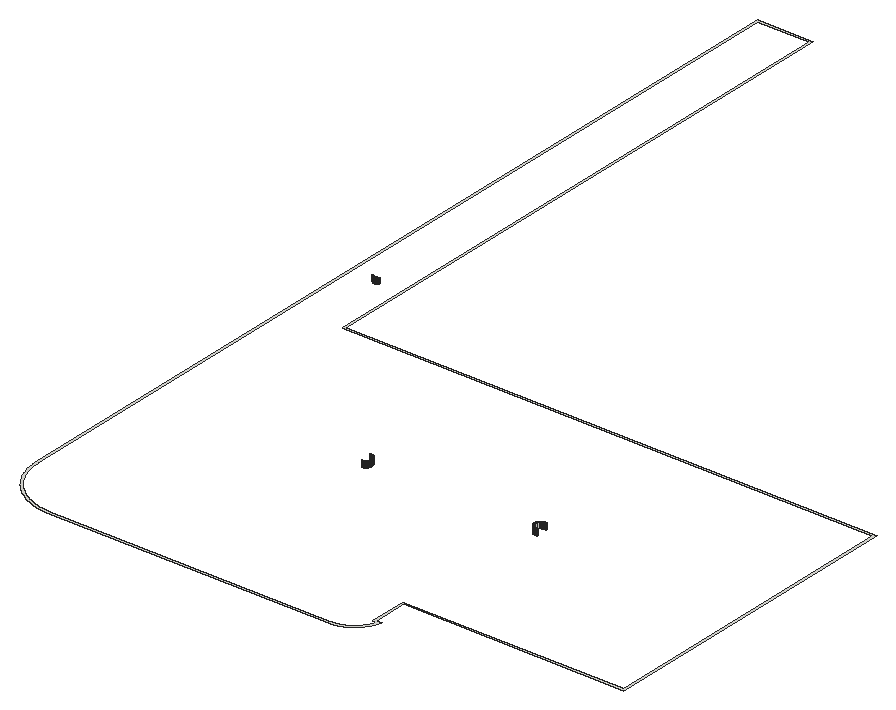
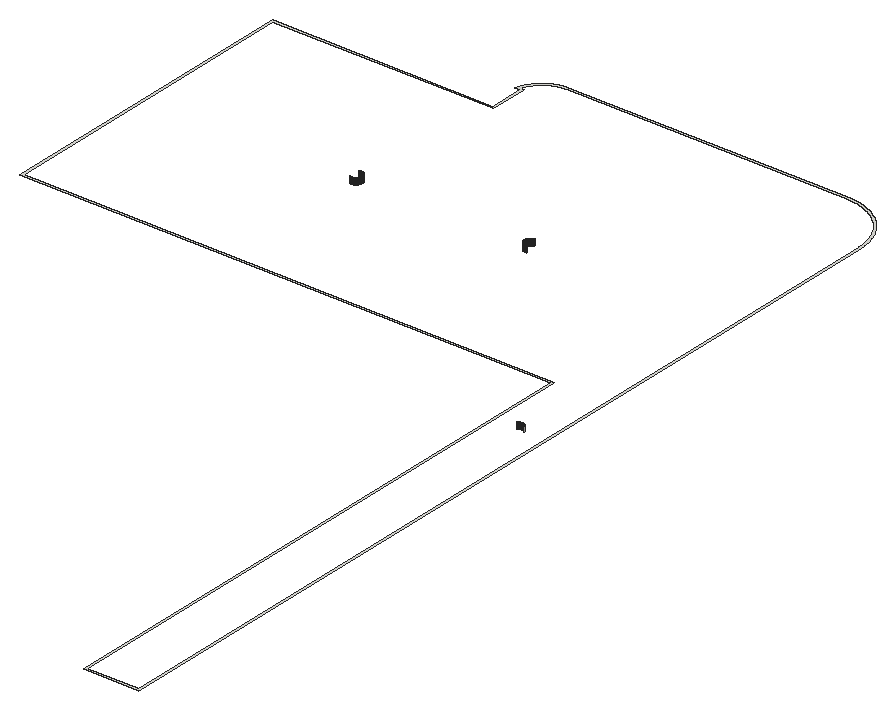
# SketchUp Ruby script. Lengths in inches.
U = 1.inch
M = Sketchup.active_model
def pt(a) = Geom::Point3d.new(a.map { |v| v * U })
def face(e, loops, mat)
  f = e.add_face(loops[0].map { |a| pt(a) })
  loops[1..].each { |l| e.add_face(l.map { |a| pt(a) }).erase! }
  f.material = f.back_material = mat if mat
  f
end
# faces: each face lists its corners as indices into pts; further lists are holes
def faces(e, pts, list, mat = nil) = list.each { |f| face(e, (f[0].is_a?(Array) ? f : [f]).map { |l| l.map { |i| pts[i] } }, mat) }
# xy, xz, yz: faces in a plane at the given z, y or x. An outline is a flat list of corners, or four numbers for a rectangle; further outlines are holes
def ring(l) = l.size == 4 ? [[l[0], l[1]], [l[2], l[1]], [l[2], l[3]], [l[0], l[3]]] : l.each_slice(2).to_a
def flat(e, list, mat, &to3) = list.each { |f| face(e, (f[0].is_a?(Array) ? f : [f]).map { |l| ring(l).map { |u, v| to3.(u, v) } }, mat) }
def xy(e, z, list, mat = nil) = flat(e, list, mat) { |x, y| [x, y, z] }
def xz(e, y, list, mat = nil) = flat(e, list, mat) { |x, z| [x, y, z] }
def yz(e, x, list, mat = nil) = flat(e, list, mat) { |y, z| [x, y, z] }
def lines(e, pts, list) = list.each { |a, b| e.add_line(pt(pts[a]), pt(pts[b])) }
# prism: a flat outline (further loops are holes) pulled along v
def prism(e, loops, v, mat = nil)
  f = face(e, loops, mat); d = Geom::Vector3d.new(v.map { |x| x * U })
  f.pushpull(f.normal.samedirection?(d) ? d.length : -d.length)
end
def box(e, o, s, mat = nil) = prism(e, [[o, [o[0] + s[0], o[1], o[2]], [o[0] + s[0], o[1] + s[1], o[2]], [o[0], o[1] + s[1], o[2]]]], [0, 0, s[2]], mat)
def at(x, y, z, deg = 0) = Geom::Transformation.translation(pt([x, y, z])) * Geom::Transformation.rotation(ORIGIN, Z_AXIS, deg.degrees)
def axes(o, x, y, z) = Geom::Transformation.new([*x, 0, *y, 0, *z, 0, *pt(o).to_a, 1])
def part(name) = M.definitions.add(name)
# library, detail: a bought-in or finely detailed component or shape, given as its bounding box
def library(name, o, s) = part(name).tap { |d| box(d.entities, o, s) }
def detail(e, o, s) = box(e.add_group.entities, o, s)
def put(e, d, t, mat = nil) = e.add_instance(d, t).tap { |i| i.material = mat if mat }
def group(e, t, mat = nil) = e.add_group.tap { |g| g.transformation = t; g.material = mat if mat }.entities
root = M.entities
xy(root,258.5,[[[43.62,68,42.86,68.02,42.48,68.04,42.1,68.0625,41.72,68.09,41.35,68.12,40.59,68.2,40.21,68.25,39.84,68.3,39.46,68.36,39.09,68.42,38.72,68.49,38.34,68.56,37.97,68.63,37.6,68.72,37.23,68.8,36.86,68.89,36.49,68.99,36.13,69.09,35.76,69.19,35.4,69.3,34.32,69.66,33.96,69.79,33.61,69.93,33.25,70.06,32.2,70.51,31.86,70.66,31.52,70.83,31.17,70.99,30.83,71.16,30.5,71.34,30.16,71.51,29.17,72.08,28.85,72.27,28.53,72.47,27.57,73.1,26.95,73.54,26.65,73.76,26.35,73.99,26.05,74.23,25.75,74.46,25.46,74.7,24.88,75.2,24.6,75.45,24.31,75.7,24.04,75.96,23.76,76.23,23.49,76.49,23.23,76.76,22.96,77.04,22.7,77.31,22.45,77.6,22.2,77.88,21.7,78.46,21.46,78.75,21.23,79.05,20.99,79.35,20.76,79.65,20.54,79.95,20.1,80.57,19.47,81.53,19.27,81.85,19.08,82.17,18.51,83.16,18.34,83.5,18.16,83.83,17.99,84.17,17.83,84.52,17.66,84.86,17.51,85.2,17.06,86.25,16.93,86.61,16.79,86.96,16.66,87.32,16.3,88.4,16.19,88.76,16.09,89.13,15.99,89.49,15.89,89.86,15.8,90.23,15.72,90.6,15.63,90.97,15.56,91.34,15.49,91.72,15.42,92.09,15.36,92.46,15.3,92.84,15.25,93.21,15.2,93.59,15.12,94.35,15.09,94.72,15.0625,95.1,15.04,95.48,15.02,95.86,15,96.62,15,551,43,551,43,257,310,257,310,98,199,98,199,81,201.52,81,201.48,80.82,201.42,80.6,201.36,80.39,201.3,80.17,201.24,79.96,201.1,79.54,201.02,79.33,200.95,79.12,200.71,78.49,200.53,78.09,200.4375,77.88,200.34,77.68,200.25,77.48,200.15,77.28,200.04,77.08,199.94,76.89,199.83,76.69,199.61,76.31,199.49,76.12,199.38,75.93,199.26,75.74,199.13,75.56,199.01,75.37,198.88,75.1875,198.75,75.01,198.49,74.65,198.35,74.48,198.21,74.3,197.93,73.96,197.78,73.79,197.48,73.46,197.18,73.14,196.86,72.82,196.54,72.52,196.21,72.22,196.04,72.07,195.7,71.79,195.52,71.65,195.35,71.51,194.99,71.25,194.8125,71.12,194.63,70.99,194.44,70.87,194.26,70.74,194.07,70.62,193.88,70.51,193.69,70.39,193.31,70.17,193.11,70.06,192.92,69.96,192.72,69.85,192.52,69.75,192.32,69.66,192.12,69.5625,191.91,69.47,191.51,69.29,190.88,69.05,190.67,68.98,190.46,68.9,190.04,68.76,189.83,68.7,189.61,68.64,189.4,68.58,189.18,68.52,188.97,68.47,188.53,68.37,188.32,68.33,188.1,68.28,187.88,68.25,187.66,68.21,187.4375,68.18,187.22,68.15,186.78,68.09,186.56,68.07,186.33,68.05,186.11,68.04,185.89,68.02,185.67,68.01,185.45,68.01,185.22,68],[43.63,69,185.21,69,185.42,69.01,185.63,69.01,186.05,69.03,186.26,69.05,186.46,69.07,186.88,69.11,187.3,69.17,187.5,69.2,187.71,69.23,187.92,69.27,188.12,69.31,188.33,69.35,188.53,69.39,188.74,69.44,188.9375,69.49,189.14,69.55,189.34,69.6,189.94,69.78,190.54,69.99,190.73,70.0625,190.93,70.14,191.12,70.22,191.32,70.3,191.51,70.38,192.08,70.65,192.26,70.74,192.45,70.84,192.63,70.9375,192.82,71.04,193,71.14,193.54,71.47,193.71,71.58,193.89,71.7,194.0625,71.8125,194.23,71.93,194.4,72.06,194.57,72.18,194.91,72.44,195.39,72.83,195.71,73.11,196.01,73.39,196.16,73.54,196.3125,73.6875,196.46,73.84,196.61,73.99,196.89,74.29,197.17,74.61,197.56,75.09,197.82,75.43,197.94,75.6,198.07,75.77,198.1875,75.9375,198.3,76.11,198.42,76.29,198.53,76.46,198.86,77,198.96,77.18,199.0625,77.37,199.16,77.55,199.26,77.74,199.35,77.92,199.62,78.49,199.7,78.68,199.78,78.88,199.86,79.07,199.9375,79.27,200.01,79.46,200.15,79.86,200.2,80,198,80,198,99,309,99,309,256,42,256,42,550,16,550,16,96.63,16.01,96.27,16.02,95.9,16.04,95.53,16.06,95.17,16.09,94.8,16.12,94.4375,16.15,94.07,16.19,93.71,16.24,93.35,16.29,92.98,16.34,92.62,16.4,92.26,16.61,91.18,16.77,90.46,16.86,90.11,16.95,89.75,17.15,89.05,17.37,88.35,17.61,87.65,17.73,87.31,17.86,86.97,17.99,86.625,18.13,86.28,18.27,85.95,18.42,85.61,18.57,85.28,19.05,84.29,19.22,83.96,19.39,83.64,19.75,83,19.9375,82.68,20.125,82.37,20.32,82.06,20.72,81.44,20.92,81.14,21.13,80.84,21.35,80.54,21.56,80.25,21.79,79.95,22.01,79.67,22.24,79.38,22.47,79.1,23.19,78.26,23.4375,77.99,23.69,77.73,23.94,77.46,24.46,76.94,24.73,76.69,24.99,76.4375,25.26,76.19,26.1,75.47,26.38,75.24,26.67,75.01,26.95,74.79,27.25,74.56,27.54,74.35,27.84,74.13,28.14,73.92,28.44,73.72,29.06,73.32,29.37,73.125,29.68,72.9375,30,72.75,30.64,72.39,30.96,72.22,31.29,72.05,32.28,71.57,32.61,71.42,32.95,71.27,33.28,71.13,33.625,70.99,33.97,70.86,34.31,70.73,34.65,70.61,35.35,70.37,36.05,70.15,36.75,69.95,37.11,69.86,37.46,69.77,38.18,69.61,39.26,69.4,39.62,69.34,39.98,69.29,40.35,69.24,40.71,69.19,41.07,69.15,41.4375,69.12,41.8,69.09,42.17,69.06,42.53,69.04,42.9,69.02,43.27,69.01]]])
xz(root,174.5,[[116.67,258,116.75,261],[116.75,258,116.82,261],[204.18,258,204.25,261],[204.25,258,204.33,261],[204.33,258,204.41,261],
  [204.41,258,204.49,261]])
xz(root,180.5,[[116.51,258,116.59,261],[116.59,258,116.67,261],[116.67,258,116.75,261],[116.75,258,116.82,261],[204.18,258,204.25,261],
  [204.25,258,204.33,261],[204.33,258,204.41,261],[204.41,258,204.49,261]])
xz(root,292.67,[[28.84,258,28.92,261],[28.92,258,29,261],[29,258,29.08,261],[29.08,258,29.16,261]])
xz(root,292.68,[[28.6875,258,28.76,261],[29.24,258,29.3125,261]])
yz(root,119.66,[[177.26,258,177.34,261],[177.66,258,177.74,261]])
yz(root,119.67,[[177.42,258,177.5,261],[177.5,258,177.58,261]])
yz(root,201.33,[[177.42,258,177.5,261],[177.5,258,177.58,261]])
yz(root,201.34,[[177.26,258,177.34,261],[177.66,258,177.74,261]])
p = [[116.9,174.51,258],[116.82,174.5,258],[116.82,174.5,261],[116.9,174.51,261],[116.98,174.52,258],[116.98,174.52,261],
  [117.06,174.53,258],[117.06,174.53,261],[117.14,174.54,258],[117.14,174.54,261],[117.21,174.55,258],[117.21,174.55,261],
  [203.86,174.54,258],[203.79,174.55,258],[203.79,174.55,261],[203.86,174.54,261],[203.94,174.53,258],[203.94,174.53,261],
  [204.02,174.52,258],[204.02,174.52,261],[204.1,174.51,258],[204.1,174.51,261],[204.18,174.5,258],[204.18,174.5,261],
  [204.57,174.51,258],[204.49,174.5,258],[204.49,174.5,261],[204.57,174.51,261],[204.65,174.52,258],[204.65,174.52,261],
  [204.72,174.53,258],[204.72,174.53,261],[204.8,174.54,258],[204.8,174.54,261],[204.88,174.55,258],[204.88,174.55,261],
  [117.29,174.57,258],[117.29,174.57,261],[117.37,174.58,258],[117.37,174.58,261],[117.44,174.6,258],[117.44,174.6,261],
  [117.52,174.625,258],[117.52,174.625,261],[117.59,174.65,258],[117.59,174.65,261],[117.67,174.67,258],[117.67,174.67,261],
  [203.41,174.65,258],[203.33,174.67,258],[203.33,174.67,261],[203.41,174.65,261],[203.48,174.625,258],[203.48,174.625,261],
  [203.56,174.6,258],[203.56,174.6,261],[203.63,174.58,258],[203.63,174.58,261],[203.71,174.57,258],[203.71,174.57,261],
  [204.96,174.57,258],[204.96,174.57,261],[205.03,174.58,258],[205.03,174.58,261],[205.11,174.6,258],[205.11,174.6,261],
  [205.19,174.625,258],[205.19,174.625,261],[205.26,174.65,258],[205.26,174.65,261],[205.33,174.67,258],[205.33,174.67,261],
  [117.74,174.7,258],[117.74,174.7,261],[117.81,174.73,258],[117.81,174.73,261],[117.89,174.76,258],[117.89,174.76,261],
  [203.19,174.73,258],[203.11,174.76,258],[203.11,174.76,261],[203.19,174.73,261],[203.26,174.7,258],[203.26,174.7,261],
  [205.41,174.7,258],[205.41,174.7,261],[117.96,174.79,258],[117.96,174.79,261],[118.03,174.83,258],[118.03,174.83,261],
  [118.1,174.86,258],[118.1,174.86,261],[202.97,174.83,258],[202.9,174.86,258],[202.9,174.86,261],[202.97,174.83,261],
  [203.04,174.79,258],[203.04,174.79,261],[118.17,174.9,258],[118.17,174.9,261],[118.23,174.94,258],[118.23,174.94,261],
  [118.3,174.98,258],[118.3,174.98,261],[202.77,174.94,258],[202.7,174.98,258],[202.7,174.98,261],[202.77,174.94,261],
  [202.83,174.9,258],[202.83,174.9,261],[118.37,175.03,258],[118.37,175.03,261],[118.43,175.07,258],[118.43,175.07,261],
  [202.63,175.03,258],[202.57,175.07,258],[202.57,175.07,261],[202.63,175.03,261],[118.49,175.12,258],[118.49,175.12,261],
  [118.55,175.17,258],[118.55,175.17,261],[202.51,175.12,258],[202.45,175.17,258],[202.45,175.17,261],[202.51,175.12,261],
  [118.62,175.22,258],[118.62,175.22,261],[118.67,175.27,258],[118.67,175.27,261],[202.38,175.22,258],[202.33,175.27,258],
  [202.33,175.27,261],[202.38,175.22,261],[118.73,175.32,258],[118.73,175.32,261],[118.79,175.38,258],[118.79,175.38,261],
  [202.27,175.32,258],[202.21,175.38,258],[202.21,175.38,261],[202.27,175.32,261],[118.84,175.43,258],[118.84,175.43,261],
  [118.9,175.49,258],[118.9,175.49,261],[202.16,175.43,258],[202.1,175.49,258],[202.1,175.49,261],[202.16,175.43,261],
  [118.95,175.55,258],[118.95,175.55,261],[202.05,175.55,258],[202.05,175.55,261],[119,175.61,258],[119,175.61,261],
  [119.05,175.67,258],[119.05,175.67,261],[202,175.61,258],[201.95,175.67,258],[201.95,175.67,261],[202,175.61,261],
  [119.09,175.74,258],[119.09,175.74,261],[119.14,175.8,258],[119.14,175.8,261],[201.91,175.74,258],[201.86,175.8,258],
  [201.86,175.8,261],[201.91,175.74,261],[119.18,175.87,258],[119.18,175.87,261],[201.82,175.87,258],[201.82,175.87,261],
  [119.22,175.93,258],[119.22,175.93,261],[119.26,176,258],[119.26,176,261],[201.78,175.93,258],[201.74,176,258],
  [201.74,176,261],[201.78,175.93,261],[119.3,176.07,258],[119.3,176.07,261],[201.7,176.07,258],[201.7,176.07,261],
  [119.34,176.14,258],[119.34,176.14,261],[119.375,176.21,258],[119.375,176.21,261],[201.66,176.14,258],[201.625,176.21,258],
  [201.625,176.21,261],[201.66,176.14,261],[119.41,176.28,258],[119.41,176.28,261],[201.59,176.28,258],[201.59,176.28,261],
  [119.4375,176.35,258],[119.4375,176.35,261],[201.5625,176.35,258],[201.5625,176.35,261],[119.47,176.42,258],[119.47,176.42,261],
  [119.49,176.5,258],[119.49,176.5,261],[201.53,176.42,258],[201.51,176.5,258],[201.51,176.5,261],[201.53,176.42,261],
  [119.52,176.57,258],[119.52,176.57,261],[201.48,176.57,258],[201.48,176.57,261],[119.54,176.65,258],[119.54,176.65,261],
  [119.5625,176.72,258],[119.5625,176.72,261],[201.46,176.65,258],[201.4375,176.72,258],[201.4375,176.72,261],[201.46,176.65,261],
  [119.58,176.8,258],[119.58,176.8,261],[201.42,176.8,258],[201.42,176.8,261],[119.6,176.875,258],[119.6,176.875,261],
  [201.4,176.875,258],[201.4,176.875,261],[119.62,176.95,258],[119.62,176.95,261],[201.38,176.95,258],[201.38,176.95,261],
  [119.63,177.03,258],[119.63,177.03,261],[119.64,177.11,258],[119.64,177.11,261],[201.37,177.03,258],[201.36,177.11,258],
  [201.36,177.11,261],[201.37,177.03,261],[119.65,177.1875,258],[119.65,177.1875,261],[201.35,177.1875,258],[201.35,177.1875,261],
  [119.66,177.26,258],[119.66,177.26,261],[201.34,177.26,258],[201.34,177.26,261],[119.67,177.42,258],[119.66,177.34,258],
  [119.66,177.34,261],[119.67,177.42,261],[201.34,177.34,258],[201.33,177.42,258],[201.33,177.42,261],[201.34,177.34,261],
  [119.66,177.66,258],[119.67,177.58,258],[119.67,177.58,261],[119.66,177.66,261],[201.33,177.58,258],[201.34,177.66,258],
  [201.34,177.66,261],[201.33,177.58,261],[119.65,177.8125,258],[119.66,177.74,258],[119.66,177.74,261],[119.65,177.8125,261],
  [201.34,177.74,258],[201.35,177.8125,258],[201.35,177.8125,261],[201.34,177.74,261],[119.64,177.89,258],[119.64,177.89,261],
  [201.36,177.89,258],[201.36,177.89,261],[119.63,177.97,258],[119.63,177.97,261],[201.37,177.97,258],[201.37,177.97,261],
  [119.6,178.125,258],[119.62,178.05,258],[119.62,178.05,261],[119.6,178.125,261],[201.38,178.05,258],[201.38,178.05,261],
  [201.4,178.125,258],[201.4,178.125,261],[119.58,178.2,258],[119.58,178.2,261],[201.42,178.2,258],[201.42,178.2,261],
  [119.5625,178.28,258],[119.5625,178.28,261],[201.4375,178.28,258],[201.4375,178.28,261],[119.54,178.35,258],[119.54,178.35,261],
  [201.46,178.35,258],[201.46,178.35,261],[119.49,178.5,258],[119.52,178.43,258],[119.52,178.43,261],[119.49,178.5,261],
  [201.48,178.43,258],[201.48,178.43,261],[201.51,178.5,258],[201.51,178.5,261],[119.47,178.58,258],[119.47,178.58,261],
  [201.53,178.58,258],[201.53,178.58,261],[119.41,178.72,258],[119.4375,178.65,258],[119.4375,178.65,261],[119.41,178.72,261],
  [201.5625,178.65,258],[201.5625,178.65,261],[201.59,178.72,258],[201.59,178.72,261],[119.375,178.79,258],[119.375,178.79,261],
  [201.625,178.79,258],[201.625,178.79,261],[119.34,178.86,258],[119.34,178.86,261],[201.66,178.86,258],[201.66,178.86,261],
  [119.26,179,258],[119.3,178.93,258],[119.3,178.93,261],[119.26,179,261],[201.7,178.93,258],[201.7,178.93,261],
  [201.74,179,258],[201.74,179,261],[119.22,179.07,258],[119.22,179.07,261],[201.78,179.07,258],[201.78,179.07,261],
  [119.14,179.2,258],[119.18,179.13,258],[119.18,179.13,261],[119.14,179.2,261],[201.82,179.13,258],[201.82,179.13,261],
  [201.86,179.2,258],[201.86,179.2,261],[119.09,179.26,258],[119.09,179.26,261],[201.91,179.26,258],[201.91,179.26,261],
  [119,179.39,258],[119.05,179.33,258],[119.05,179.33,261],[119,179.39,261],[201.95,179.33,258],[201.95,179.33,261],
  [202,179.39,258],[202,179.39,261],[118.9,179.51,258],[118.95,179.45,258],[118.95,179.45,261],[118.9,179.51,261],
  [202.05,179.45,258],[202.05,179.45,261],[202.1,179.51,258],[202.1,179.51,261],[118.84,179.57,258],[118.84,179.57,261],
  [202.16,179.57,258],[202.16,179.57,261],[118.73,179.68,258],[118.79,179.62,258],[118.79,179.62,261],[118.73,179.68,261],
  [202.21,179.62,258],[202.21,179.62,261],[202.27,179.68,258],[202.27,179.68,261],[118.62,179.78,258],[118.67,179.73,258],
  [118.67,179.73,261],[118.62,179.78,261],[202.33,179.73,258],[202.33,179.73,261],[202.38,179.78,258],[202.38,179.78,261],
  [118.49,179.88,258],[118.55,179.83,258],[118.55,179.83,261],[118.49,179.88,261],[202.45,179.83,258],[202.45,179.83,261],
  [202.51,179.88,258],[202.51,179.88,261],[118.37,179.97,258],[118.43,179.93,258],[118.43,179.93,261],[118.37,179.97,261],
  [202.57,179.93,258],[202.57,179.93,261],[202.63,179.97,258],[202.63,179.97,261],[118.23,180.06,258],[118.3,180.02,258],
  [118.3,180.02,261],[118.23,180.06,261],[202.7,180.02,258],[202.7,180.02,261],[202.77,180.06,258],[202.77,180.06,261],
  [118.03,180.17,258],[118.1,180.14,258],[118.1,180.14,261],[118.03,180.17,261],[118.17,180.1,258],[118.17,180.1,261],
  [202.83,180.1,258],[202.83,180.1,261],[202.9,180.14,258],[202.9,180.14,261],[202.97,180.17,258],[202.97,180.17,261],
  [117.81,180.27,258],[117.89,180.24,258],[117.89,180.24,261],[117.81,180.27,261],[117.96,180.21,258],[117.96,180.21,261],
  [203.04,180.21,258],[203.04,180.21,261],[203.11,180.24,258],[203.11,180.24,261],[203.19,180.27,258],[203.19,180.27,261],
  [117.59,180.35,258],[117.67,180.33,258],[117.67,180.33,261],[117.59,180.35,261],[117.74,180.3,258],[117.74,180.3,261],
  [203.26,180.3,258],[203.26,180.3,261],[203.33,180.33,258],[203.33,180.33,261],[203.41,180.35,258],[203.41,180.35,261],
  [205.26,180.35,258],[205.33,180.33,258],[205.33,180.33,261],[205.26,180.35,261],[116.04,180.43,258],[116.12,180.45,258],
  [116.12,180.45,261],[116.04,180.43,261],[116.2,180.46,258],[116.2,180.46,261],[117.14,180.46,258],[117.21,180.45,258],
  [117.21,180.45,261],[117.14,180.46,261],[117.29,180.43,258],[117.29,180.43,261],[117.37,180.42,258],[117.37,180.42,261],
  [117.44,180.4,258],[117.44,180.4,261],[117.52,180.375,258],[117.52,180.375,261],[203.48,180.375,258],[203.48,180.375,261],
  [203.56,180.4,258],[203.56,180.4,261],[203.63,180.42,258],[203.63,180.42,261],[203.71,180.43,258],[203.71,180.43,261],
  [203.79,180.45,258],[203.79,180.45,261],[203.86,180.46,258],[203.86,180.46,261],[204.8,180.46,258],[204.88,180.45,258],
  [204.88,180.45,261],[204.8,180.46,261],[204.96,180.43,258],[204.96,180.43,261],[205.03,180.42,258],[205.03,180.42,261],
  [205.11,180.4,258],[205.11,180.4,261],[205.19,180.375,258],[205.19,180.375,261],[116.28,180.47,258],[116.28,180.47,261],
  [116.35,180.48,258],[116.35,180.48,261],[116.43,180.49,258],[116.43,180.49,261],[116.51,180.5,258],[116.51,180.5,261],
  [116.82,180.5,258],[116.9,180.49,258],[116.9,180.49,261],[116.82,180.5,261],[116.98,180.48,258],[116.98,180.48,261],
  [117.06,180.47,258],[117.06,180.47,261],[203.94,180.47,258],[203.94,180.47,261],[204.02,180.48,258],[204.02,180.48,261],
  [204.1,180.49,258],[204.1,180.49,261],[204.18,180.5,258],[204.18,180.5,261],[204.49,180.5,258],[204.57,180.49,258],
  [204.57,180.49,261],[204.49,180.5,261],[204.65,180.48,258],[204.65,180.48,261],[204.72,180.47,258],[204.72,180.47,261],
  [28.3,292.75,258],[28.22,292.77,258],[28.22,292.77,261],[28.3,292.75,261],[28.375,292.73,258],[28.375,292.73,261],
  [28.45,292.72,258],[28.45,292.72,261],[28.53,292.7,258],[28.53,292.7,261],[28.61,292.69,258],[28.61,292.69,261],
  [28.6875,292.68,258],[28.6875,292.68,261],[28.84,292.67,258],[28.76,292.68,258],[28.76,292.68,261],[28.84,292.67,261],
  [29.24,292.68,258],[29.16,292.67,258],[29.16,292.67,261],[29.24,292.68,261],[29.39,292.69,258],[29.3125,292.68,258],
  [29.3125,292.68,261],[29.39,292.69,261],[29.47,292.7,258],[29.47,292.7,261],[29.55,292.72,258],[29.55,292.72,261],
  [29.625,292.73,258],[29.625,292.73,261],[29.7,292.75,258],[29.7,292.75,261],[29.78,292.77,258],[29.78,292.77,261],
  [28,292.84,258],[27.92,292.87,258],[27.92,292.87,261],[28,292.84,261],[28.07,292.8125,258],[28.07,292.8125,261],
  [28.15,292.79,258],[28.15,292.79,261],[29.85,292.79,258],[29.85,292.79,261],[29.93,292.8125,258],[29.93,292.8125,261],
  [30,292.84,258],[30,292.84,261],[30.08,292.87,258],[30.08,292.87,261],[27.78,292.93,258],[27.71,292.96,258],
  [27.71,292.96,261],[27.78,292.93,261],[27.85,292.9,258],[27.85,292.9,261],[30.15,292.9,258],[30.15,292.9,261],
  [30.22,292.93,258],[30.22,292.93,261],[30.29,292.96,258],[30.29,292.96,261],[27.57,293.03,258],[27.5,293.07,258],
  [27.5,293.07,261],[27.57,293.03,261],[27.64,292.99,258],[27.64,292.99,261],[30.36,292.99,258],[30.36,292.99,261],
  [30.43,293.03,258],[30.43,293.03,261],[30.5,293.07,258],[30.5,293.07,261],[27.43,293.11,258],[27.37,293.15,258],
  [27.37,293.15,261],[27.43,293.11,261],[30.57,293.11,258],[30.57,293.11,261],[30.63,293.15,258],[30.63,293.15,261],
  [27.24,293.24,258],[27.17,293.29,258],[27.17,293.29,261],[27.24,293.24,261],[27.3,293.19,258],[27.3,293.19,261],
  [30.7,293.19,258],[30.7,293.19,261],[30.76,293.24,258],[30.76,293.24,261],[30.83,293.29,258],[30.83,293.29,261],
  [27.11,293.34,258],[27.05,293.39,258],[27.05,293.39,261],[27.11,293.34,261],[30.89,293.34,258],[30.89,293.34,261],
  [30.95,293.39,258],[30.95,293.39,261],[26.99,293.4375,258],[26.99,293.4375,261],[31.01,293.4375,258],[31.01,293.4375,261]]
faces(root,p,[[0,1,2,3],[4,0,3,5],[6,4,5,7],[8,6,7,9],[10,8,9,11],[12,13,14,15],[16,12,15,17],[18,16,17,19],
  [20,18,19,21],[22,20,21,23],[24,25,26,27],[28,24,27,29],[30,28,29,31],[32,30,31,33],[34,32,33,35],[36,10,11,37],
  [38,36,37,39],[40,38,39,41],[42,40,41,43],[44,42,43,45],[46,44,45,47],[48,49,50,51],[52,48,51,53],[54,52,53,55],
  [56,54,55,57],[58,56,57,59],[13,58,59,14],[60,34,35,61],[62,60,61,63],[64,62,63,65],[66,64,65,67],[68,66,67,69],
  [70,68,69,71],[72,46,47,73],[74,72,73,75],[76,74,75,77],[78,79,80,81],[82,78,81,83],[49,82,83,50],[84,70,71,85],
  [86,76,77,87],[88,86,87,89],[90,88,89,91],[92,93,94,95],[96,92,95,97],[79,96,97,80],[98,90,91,99],[100,98,99,101],
  [102,100,101,103],[104,105,106,107],[108,104,107,109],[93,108,109,94],[110,102,103,111],[112,110,111,113],[114,115,116,117],[105,114,117,106],
  [118,112,113,119],[120,118,119,121],[122,123,124,125],[115,122,125,116],[126,120,121,127],[128,126,127,129],[130,131,132,133],[123,130,133,124],
  [134,128,129,135],[136,134,135,137],[138,139,140,141],[131,138,141,132],[142,136,137,143],[144,142,143,145],[146,147,148,149],[139,146,149,140],
  [150,144,145,151],[147,152,153,148],[154,150,151,155],[156,154,155,157],[158,159,160,161],[152,158,161,153],[162,156,157,163],[164,162,163,165],
  [166,167,168,169],[159,166,169,160],[170,164,165,171],[167,172,173,168],[174,170,171,175],[176,174,175,177],[178,179,180,181],[172,178,181,173],
  [182,176,177,183],[179,184,185,180],[186,182,183,187],[188,186,187,189],[190,191,192,193],[184,190,193,185],[194,188,189,195],[191,196,197,192],
  [198,194,195,199],[196,200,201,197],[202,198,199,203],[204,202,203,205],[206,207,208,209],[200,206,209,201],[210,204,205,211],[207,212,213,208],
  [214,210,211,215],[216,214,215,217],[218,219,220,221],[212,218,221,213],[222,216,217,223],[219,224,225,220],[226,222,223,227],[224,228,229,225],
  [230,226,227,231],[228,232,233,229],[234,230,231,235],[236,234,235,237],[238,239,240,241],[232,238,241,233],[242,236,237,243],[239,244,245,240],
  [246,242,243,247],[244,248,249,245],[250,251,252,253],[254,255,256,257],[258,259,260,261],[262,263,264,265],[266,267,268,269],[270,271,272,273],
  [274,266,269,275],[271,276,277,272],[278,274,275,279],[276,280,281,277],[282,283,284,285],[283,278,279,284],[280,286,287,281],[286,288,289,287],
  [290,282,285,291],[288,292,293,289],[294,290,291,295],[292,296,297,293],[298,294,295,299],[296,300,301,297],[302,303,304,305],[303,298,299,304],
  [300,306,307,301],[306,308,309,307],[310,302,305,311],[308,312,313,309],[314,315,316,317],[315,310,311,316],[312,318,319,313],[318,320,321,319],
  [322,314,317,323],[320,324,325,321],[326,322,323,327],[324,328,329,325],[330,331,332,333],[331,326,327,332],[328,334,335,329],[334,336,337,335],
  [338,330,333,339],[336,340,341,337],[342,343,344,345],[343,338,339,344],[340,346,347,341],[346,348,349,347],[350,342,345,351],[348,352,353,349],
  [354,355,356,357],[355,350,351,356],[352,358,359,353],[358,360,361,359],[362,363,364,365],[363,354,357,364],[360,366,367,361],[366,368,369,367],
  [370,362,365,371],[368,372,373,369],[374,375,376,377],[375,370,371,376],[372,378,379,373],[378,380,381,379],[382,383,384,385],[383,374,377,384],
  [380,386,387,381],[386,388,389,387],[390,391,392,393],[391,382,385,392],[388,394,395,389],[394,396,397,395],[398,399,400,401],[399,390,393,400],
  [396,402,403,397],[402,404,405,403],[406,407,408,409],[407,398,401,408],[404,410,411,405],[410,412,413,411],[414,415,416,417],[415,418,419,416],
  [418,406,409,419],[412,420,421,413],[420,422,423,421],[422,424,425,423],[426,427,428,429],[427,430,431,428],[430,414,417,431],[424,432,433,425],
  [432,434,435,433],[434,436,437,435],[438,439,440,441],[439,442,443,440],[442,426,429,443],[436,444,445,437],[444,446,447,445],[446,448,449,447],
  [450,451,452,453],[454,455,456,457],[455,458,459,456],[460,461,462,463],[461,464,465,462],[464,466,467,465],[466,468,469,467],[468,470,471,469],
  [470,438,441,471],[448,472,473,449],[472,474,475,473],[474,476,477,475],[476,478,479,477],[478,480,481,479],[480,482,483,481],[484,485,486,487],
  [485,488,489,486],[488,490,491,489],[490,492,493,491],[492,494,495,493],[494,450,453,495],[458,496,497,459],[496,498,499,497],[498,500,501,499],
  [500,502,503,501],[504,505,506,507],[505,508,509,506],[508,510,511,509],[510,460,463,511],[482,512,513,483],[512,514,515,513],[514,516,517,515],
  [516,518,519,517],[520,521,522,523],[521,524,525,522],[524,526,527,525],[526,484,487,527],[528,529,530,531],[532,528,531,533],[534,532,533,535],
  [536,534,535,537],[538,536,537,539],[540,538,539,541],[542,543,544,545],[546,547,548,549],[550,551,552,553],[554,550,553,555],[556,554,555,557],
  [558,556,557,559],[560,558,559,561],[562,560,561,563],[564,565,566,567],[568,564,567,569],[570,568,569,571],[529,570,571,530],[572,562,563,573],
  [574,572,573,575],[576,574,575,577],[578,576,577,579],[580,581,582,583],[584,580,583,585],[565,584,585,566],[586,578,579,587],[588,586,587,589],
  [590,588,589,591],[592,593,594,595],[596,592,595,597],[581,596,597,582],[598,590,591,599],[600,598,599,601],[602,600,601,603],[604,605,606,607],
  [593,604,607,594],[608,602,603,609],[610,608,609,611],[612,613,614,615],[616,612,615,617],[605,616,617,606],[618,610,611,619],[620,618,619,621],
  [622,620,621,623],[624,625,626,627],[613,624,627,614],[628,622,623,629],[630,628,629,631],[625,632,633,626],[634,630,631,635]])
